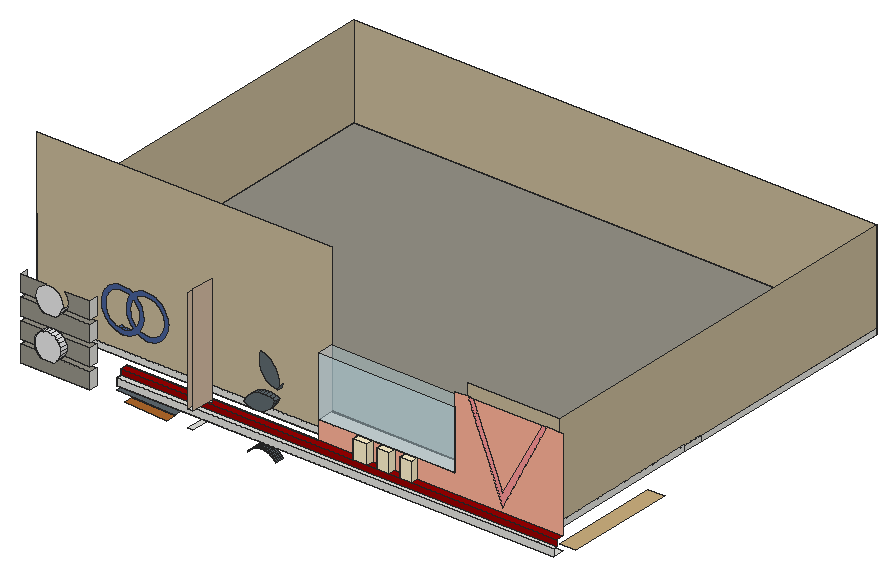
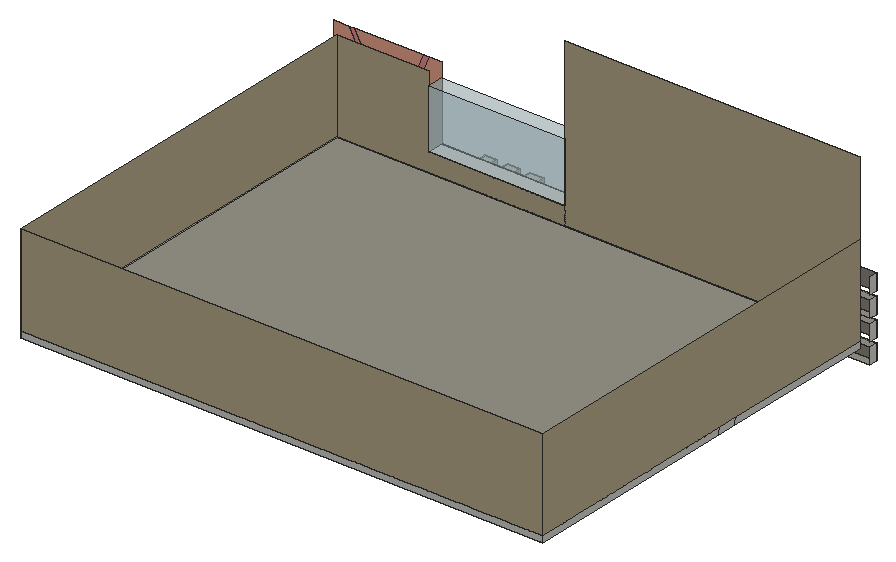
# SketchUp Ruby script. Lengths in inches.
U = 1.inch
M = Sketchup.active_model
def pt(a) = Geom::Point3d.new(a.map { |v| v * U })
def face(e, loops, mat)
  f = e.add_face(loops[0].map { |a| pt(a) })
  loops[1..].each { |l| e.add_face(l.map { |a| pt(a) }).erase! }
  f.material = f.back_material = mat if mat
  f
end
# faces: each face lists its corners as indices into pts; further lists are holes
def faces(e, pts, list, mat = nil) = list.each { |f| face(e, (f[0].is_a?(Array) ? f : [f]).map { |l| l.map { |i| pts[i] } }, mat) }
# xy, xz, yz: faces in a plane at the given z, y or x. An outline is a flat list of corners, or four numbers for a rectangle; further outlines are holes
def ring(l) = l.size == 4 ? [[l[0], l[1]], [l[2], l[1]], [l[2], l[3]], [l[0], l[3]]] : l.each_slice(2).to_a
def flat(e, list, mat, &to3) = list.each { |f| face(e, (f[0].is_a?(Array) ? f : [f]).map { |l| ring(l).map { |u, v| to3.(u, v) } }, mat) }
def xy(e, z, list, mat = nil) = flat(e, list, mat) { |x, y| [x, y, z] }
def xz(e, y, list, mat = nil) = flat(e, list, mat) { |x, z| [x, y, z] }
def yz(e, x, list, mat = nil) = flat(e, list, mat) { |y, z| [x, y, z] }
def lines(e, pts, list) = list.each { |a, b| e.add_line(pt(pts[a]), pt(pts[b])) }
# prism: a flat outline (further loops are holes) pulled along v
def prism(e, loops, v, mat = nil)
  f = face(e, loops, mat); d = Geom::Vector3d.new(v.map { |x| x * U })
  f.pushpull(f.normal.samedirection?(d) ? d.length : -d.length)
end
def box(e, o, s, mat = nil) = prism(e, [[o, [o[0] + s[0], o[1], o[2]], [o[0] + s[0], o[1] + s[1], o[2]], [o[0], o[1] + s[1], o[2]]]], [0, 0, s[2]], mat)
def at(x, y, z, deg = 0) = Geom::Transformation.translation(pt([x, y, z])) * Geom::Transformation.rotation(ORIGIN, Z_AXIS, deg.degrees)
def axes(o, x, y, z) = Geom::Transformation.new([*x, 0, *y, 0, *z, 0, *pt(o).to_a, 1])
def part(name) = M.definitions.add(name)
# library, detail: a bought-in or finely detailed component or shape, given as its bounding box
def library(name, o, s) = part(name).tap { |d| box(d.entities, o, s) }
def detail(e, o, s) = box(e.add_group.entities, o, s)
def put(e, d, t, mat = nil) = e.add_instance(d, t).tap { |i| i.material = mat if mat }
def group(e, t, mat = nil) = e.add_group.tap { |g| g.transformation = t; g.material = mat if mat }.entities
root = M.entities
M.materials.add("[Color A02]").color = [255, 153, 153]
M.materials.add("[Color A07]").color = [153, 0, 0]
M.materials.add("[Color B02]").color = [255, 178, 153]
M.materials.add("[Color D01]").color = [255, 242, 204]
M.materials.add("[Formica Blue]").color = [71, 97, 152]
M.materials.add("[Formica Graystone]").color = [149, 146, 135]
M.materials.add("[Formica Laminate Light]").color = [213, 189, 164]
M.materials.add("[Formica Speckled Grey]").color = [94, 105, 111]
M.materials.add("[Polished Concrete Old]").color = [229, 229, 229]
M.materials.add("[Quartz Light Brown]").color = [199, 184, 152]
M.materials.add("[Translucent Glass Safety]").color = [204, 235, 244]
M.materials["[Translucent Glass Safety]"].alpha = 0.5
M.materials.add("[Wood Bamboo]").color = [177, 105, 43]
M.materials.add("[Wood Floor Light]").color = [204, 176, 127]
xy(root,237.71,[[205.21,257.39,307.34,269.01]],"[Formica Graystone]")
xy(root,241.92,[[424.62,250.56,360.2,253.39,360.79,266.8125,425.21,263.99]],"[Wood Bamboo]")
xy(root,242.2,[[724.72,520.41,868.85,550.03]])
xy(root,251.7,[[963.43,293.12,987.53,454.16]],"[Wood Floor Light]")
xy(root,253.37,[[436.06,250.0625,436.64,263.49,349.35,267.3125,348.76,253.89]],"[Formica Speckled Grey]")
xy(root,258.72,[[479.36,228.58,480.8,261.55,473.4,261.88,471.96,228.91]])
xy(root,259.36,[[491.29,256.01,630.73,269.01]])
xy(root,261.0625,[[963.43,252.2,987.53,269.01]])
xy(root,261.0625,[[350.6,252.2,350.6,269.01,630.73,269.01,630.73,293.12,963.43,293.12,963.43,252.2]],"[Formica Graystone]")
xy(root,261.71,[[205.21,257.39,307.34,269.01]],"[Formica Graystone]")
xy(root,261.71,[[246.96,246.45,260.84,257.39]],"[Polished Concrete Old]")
xy(root,271.3125,[[350.6,252.2,963.43,258.7],[963.43,252.2,987.53,258.7],[350.6,258.7,350.6,269.01,630.73,269.01,630.73,293.12,963.43,293.12,963.43,258.7],[200.82,520.41,963.43,550.03],[200.82,550.03,963.43,870.85]])
xy(root,271.3125,[[200.82,293.12,963.43,520.41]],"[Formica Graystone]")
xy(root,280.3125,[[350.6,258.7,689.3,269.01],[709.64,258.7,724.04,269.01],[742.55,258.7,757.83,269.01],[774.67,258.7,987.53,269.01]],"[Color A07]")
xy(root,280.3125,[[200.82,293.12,963.43,870.85]],"[Formica Graystone]")
xy(root,283.43,[[479.36,228.58,471.96,228.91,473.4,261.88,480.8,261.55]])
xy(root,292.33,[[205.21,257.39,307.34,269.01]],"[Formica Graystone]")
xy(root,298.96,[[205.21,257.39,307.34,269.01]],"[Formica Graystone]")
xy(root,307.55,[[630.73,269.01,829.97,293.12]])
xy(root,307.55,[[689.3,258.7,709.64,269.01],[724.04,258.7,742.55,269.01],[757.83,258.7,774.67,269.01]],"[Color D01]")
xy(root,318.84,[[556.52,261.14,561.09,269.01]],"[Formica Speckled Grey]")
xy(root,322.96,[[205.21,257.39,307.34,269.01]],"[Formica Graystone]")
xy(root,322.96,[[248.17,246.45,264.38,257.39]],"[Polished Concrete Old]")
xz(root,246.45,[[246.96,261.71,260.84,261.71,263.58,262.84,267.59,265.92,269.4375,268.33,270.66,269.93,272.59,274.6,273.25,279.61,272.59,284.61,270.66,289.28,268.32,292.33,267.59,293.29,263.58,296.37,258.91,298.3,253.9,298.96,248.89,298.3,244.22,296.37,240.21,293.29,239.48,292.33,237.14,289.28,235.21,284.61,234.55,279.61,235.21,274.6,237.14,269.93,238.36,268.33,240.21,265.92,244.22,262.84],[248.17,322.96,264.38,322.96,266.07,323.66,270.125,326.77,272.28,329.58,273.24,330.83,275.19,335.55,275.86,340.62,275.19,345.69,273.24,350.42,270.81,353.58,270.125,354.47,266.07,357.59,261.34,359.54,256.27,360.21,251.2,359.54,246.48,357.59,242.42,354.47,241.74,353.58,239.3125,350.42,237.35,345.69,236.6875,340.62,237.35,335.55,239.3125,330.83,240.27,329.58,242.42,326.77,246.48,323.66]],"[Polished Concrete Old]")
xz(root,252.2,[[350.6,261.0625,987.53,271.3125]])
xz(root,257.39,[[253.9,260.25,258.91,260.91,260.84,261.71,246.96,261.71,248.89,260.91],[239.48,292.33,240.21,293.29,244.22,296.37,248.89,298.3,253.9,298.96,258.91,298.3,263.58,296.37,267.59,293.29,268.32,292.33],[256.27,321.04,261.34,321.7,264.38,322.96,248.17,322.96,251.2,321.7]])
xz(root,257.39,[[205.21,237.71,307.34,237.71,307.34,261.71,260.84,261.71,258.91,260.91,253.9,260.25,248.89,260.91,246.96,261.71,205.21,261.71],[205.21,268.33,238.36,268.33,237.14,269.93,235.21,274.6,234.55,279.61,235.21,284.61,237.14,289.28,239.48,292.33,205.21,292.33],[269.4375,268.33,307.34,268.33,307.34,292.33,268.32,292.33,270.66,289.28,272.59,284.61,273.25,279.61,272.59,274.6,270.66,269.93],[205.21,298.96,307.34,298.96,307.34,322.96,264.38,322.96,261.34,321.7,256.27,321.04,251.2,321.7,248.17,322.96,205.21,322.96],[205.21,329.58,240.27,329.58,239.3125,330.83,237.35,335.55,236.6875,340.62,237.35,345.69,239.3125,350.42,241.74,353.58,205.21,353.58],
  [272.28,329.58,307.34,329.58,307.34,353.58,270.81,353.58,273.24,350.42,275.19,345.69,275.86,340.62,275.19,335.55,273.24,330.83]],"[Formica Graystone]")
xz(root,258.7,[[350.6,271.3125,987.53,280.3125]],"[Color A07]")
xz(root,258.7,[[689.3,280.3125,709.64,307.55],[724.04,280.3125,742.55,307.55],[757.83,280.3125,774.67,307.55]],"[Color D01]")
xz(root,261.14,[[545.83,293.67,550.5625,294.15,555.16,295.36,559.51,297.28,563.5,299.84,567.05,303,570.07,306.68,572.47,310.77,574.21,315.2,570.02,317,565.61,318.22,561.09,318.84,556.52,318.84,551.99,318.23,547.59,317.02,543.39,315.23,539.47,312.89,535.9,310.04,532.74,306.74,530.06,303.04,527.89,299.02,532.01,296.64,536.44,294.93,541.09,293.93],[577.86,330.87,578.89,335.32,579.32,339.87,579.125,344.43,578.32,348.93,576.92,353.28,574.95,357.4,572.4375,361.21,569.4375,364.66,566,367.67,562.19,370.19,558.08,372.18,553.74,373.59,552.125,369.125,551.23,364.46,551.07,359.71,551.65,354.99,552.96,350.42,554.97,346.12,557.62,342.17,560.86,338.69,564.59,335.76,568.74,333.44,573.2,331.8]],"[Formica Speckled Grey]")
xz(root,269.01,[[350.6,271.3125,630.73,280.3125]])
xz(root,269.01,[[900.03,286.39,963.43,414.1875,957.83,414.1875,900.03,306.49,897.72,312.17,856.24,414.1875,848.44,414.1875]],"[Color A02]")
xz(root,269.01,[[630.73,280.3125,689.3,307.55],[709.64,280.3125,724.04,307.55],[742.55,280.3125,757.83,307.55],[774.67,280.3125,987.53,280.3125,987.53,414.1875,963.43,414.1875,900.03,286.39,848.44,414.1875,829.97,414.1875,829.97,307.55,774.67,307.55],[900.03,306.49,957.83,414.1875,856.24,414.1875,897.72,312.17]],"[Color B02]")
xz(root,269.01,[[630.73,307.55,829.97,394.11]],"[Translucent Glass Safety]")
xz(root,293.12,[[200.82,271.3125,630.73,280.3125],[630.73,271.3125,963.43,280.3125]])
xz(root,293.12,[[630.73,261.0625,963.43,271.3125]],"[Formica Graystone]")
xz(root,293.12,[[200.82,280.3125,630.73,522.12],[630.73,280.3125,630.73,307.55,829.97,307.55,829.97,414.1875,963.43,414.1875,963.43,280.3125]],"[Quartz Light Brown]")
xz(root,293.12,[[630.73,307.55,829.97,394.11]],"[Translucent Glass Safety]")
xz(root,870.85,[[200.82,271.3125,963.43,280.3125]])
xz(root,870.85,[[200.82,280.3125,963.43,414.1875]],"[Quartz Light Brown]")
yz(root,200.82,[[293.12,271.3125,520.41,280.3125],[520.41,271.3125,550.03,280.3125],[550.03,271.3125,870.85,280.3125]])
yz(root,200.82,[[293.12,280.3125,870.85,414.1875]],"[Quartz Light Brown]")
yz(root,205.21,[[257.39,237.71,269.01,261.71],[257.39,268.33,269.01,292.33],[257.39,298.96,269.01,322.96],[257.39,329.58,269.01,353.58]])
yz(root,307.34,[[257.39,237.71,269.01,261.71],[257.39,268.33,269.01,292.33],[257.39,298.96,269.01,322.96],[257.39,329.58,269.01,353.58]])
yz(root,350.6,[[252.2,261.0625,269.01,271.3125],[258.7,271.3125,269.01,280.3125]])
yz(root,630.73,[[269.01,271.3125,293.12,280.3125],[269.01,307.55,293.12,394.11]])
yz(root,689.3,[[258.7,280.3125,269.01,307.55]],"[Color D01]")
yz(root,709.64,[[258.7,280.3125,269.01,307.55]],"[Color D01]")
yz(root,724.04,[[258.7,280.3125,269.01,307.55]],"[Color D01]")
yz(root,742.55,[[258.7,280.3125,269.01,307.55]],"[Color D01]")
yz(root,757.83,[[258.7,280.3125,269.01,307.55]],"[Color D01]")
yz(root,774.67,[[258.7,280.3125,269.01,307.55]],"[Color D01]")
yz(root,829.97,[[269.01,307.55,293.12,394.11]])
yz(root,963.43,[[293.12,271.3125,520.41,280.3125],[520.41,271.3125,550.03,280.3125],[550.03,271.3125,870.85,280.3125]])
yz(root,963.43,[[293.12,280.3125,870.85,414.1875]],"[Quartz Light Brown]")
p = [[537.87,269.01,238.18],[538.6,269.01,239.24],[538.6,256.01,239.24],[537.87,256.01,238.18],[578.55,269.01,239.24],[579.28,269.01,238.18],
  [579.28,256.01,238.18],[578.55,256.01,239.24],[539.39,269.01,240.27],[539.39,256.01,240.27],[577.76,269.01,240.27],[577.76,256.01,240.27],
  [540.23,269.01,241.25],[540.23,256.01,241.25],[576.92,269.01,241.25],[576.92,256.01,241.25],[541.12,269.01,242.1875],[541.12,256.01,242.1875],
  [576.03,269.01,242.1875],[576.03,256.01,242.1875],[542.06,269.01,243.08],[542.06,256.01,243.08],[575.1,269.01,243.08],[575.1,256.01,243.08],
  [543.04,269.01,243.92],[543.04,256.01,243.92],[574.11,269.01,243.92],[574.11,256.01,243.92],[544.07,269.01,244.7],[544.07,256.01,244.7],
  [573.09,269.01,244.7],[573.09,256.01,244.7],[545.13,269.01,245.4375],[545.13,256.01,245.4375],[572.02,269.01,245.4375],[572.02,256.01,245.4375],
  [546.23,269.01,246.11],[546.23,256.01,246.11],[570.92,269.01,246.11],[570.92,256.01,246.11],[547.37,269.01,246.73],[547.37,256.01,246.73],
  [569.79,269.01,246.73],[569.79,256.01,246.73],[548.54,269.01,247.28],[548.54,256.01,247.28],[568.62,269.01,247.28],[568.62,256.01,247.28],
  [549.73,269.01,247.78],[549.73,256.01,247.78],[567.42,269.01,247.78],[567.42,256.01,247.78],[550.95,269.01,248.21],[550.95,256.01,248.21],
  [566.21,269.01,248.21],[566.21,256.01,248.21],[552.1875,269.01,248.58],[552.1875,256.01,248.58],[564.97,269.01,248.58],[564.97,256.01,248.58],
  [553.44,269.01,248.88],[553.44,256.01,248.88],[563.71,269.01,248.88],[563.71,256.01,248.88],[554.72,269.01,249.11],[554.72,256.01,249.11],
  [562.4375,269.01,249.11],[562.4375,256.01,249.11],[556,269.01,249.28],[556,256.01,249.28],[561.16,269.01,249.28],[561.16,256.01,249.28],
  [557.29,269.01,249.38],[557.29,256.01,249.38],[559.87,269.01,249.38],[559.87,256.01,249.38],[558.58,269.01,249.42],[558.58,256.01,249.42],
  [473.4,261.88,283.43],[473.4,261.88,258.72],[480.8,261.55,258.72],[480.8,261.55,283.43],[244.22,257.39,262.84],[246.96,257.39,261.71],
  [246.96,246.45,261.71],[244.22,246.45,262.84],[260.84,257.39,261.71],[263.58,257.39,262.84],[263.58,246.45,262.84],[260.84,246.45,261.71],
  [240.21,257.39,265.92],[240.21,246.45,265.92],[267.59,257.39,265.92],[267.59,246.45,265.92],[238.36,257.39,268.33],[238.36,246.45,268.33],
  [269.4375,257.39,268.33],[269.4375,246.45,268.33],[237.14,257.39,269.93],[237.14,246.45,269.93],[270.66,257.39,269.93],[270.66,246.45,269.93],
  [235.21,257.39,274.6],[235.21,246.45,274.6],[272.59,257.39,274.6],[272.59,246.45,274.6],[234.55,257.39,279.61],[234.55,246.45,279.61],
  [273.25,257.39,279.61],[273.25,246.45,279.61],[235.21,257.39,284.61],[235.21,246.45,284.61],[272.59,257.39,284.61],[272.59,246.45,284.61],
  [480.8,261.55,442.52],[479.36,228.58,442.52],[479.36,228.58,283.43],[473.4,261.88,435.11],[471.96,228.91,283.43],[471.96,228.91,435.11],
  [237.14,257.39,289.28],[237.14,246.45,289.28],[270.66,257.39,289.28],[270.66,246.45,289.28],[240.21,257.39,293.29],[239.48,257.39,292.33],
  [239.48,246.45,292.33],[240.21,246.45,293.29],[268.32,257.39,292.33],[267.59,257.39,293.29],[267.59,246.45,293.29],[268.32,246.45,292.33],
  [244.22,257.39,296.37],[244.22,246.45,296.37],[263.58,257.39,296.37],[263.58,246.45,296.37],[541.09,269.01,293.93],[545.83,269.01,293.67],
  [545.83,261.14,293.67],[541.09,261.14,293.93],[550.5625,269.01,294.15],[550.5625,261.14,294.15],[536.44,269.01,294.93],[536.44,261.14,294.93],
  [555.16,269.01,295.36],[555.16,261.14,295.36],[532.01,269.01,296.64],[532.01,261.14,296.64],[559.51,269.01,297.28],[559.51,261.14,297.28],
  [248.89,257.39,298.3],[248.89,246.45,298.3],[258.91,257.39,298.3],[258.91,246.45,298.3],[527.89,269.01,299.02],[527.89,261.14,299.02],
  [563.5,269.01,299.84],[563.5,261.14,299.84],[253.9,257.39,298.96],[253.9,246.45,298.96],[530.06,269.01,303.04],[530.06,261.14,303.04],
  [567.05,269.01,303],[567.05,261.14,303],[532.74,269.01,306.74],[532.74,261.14,306.74],[570.07,269.01,306.68],[570.07,261.14,306.68],
  [535.9,269.01,310.04],[535.9,261.14,310.04],[572.47,269.01,310.77],[572.47,261.14,310.77],[539.47,269.01,312.89],[539.47,261.14,312.89],
  [574.21,269.01,315.2],[574.21,261.14,315.2],[543.39,269.01,315.23],[543.39,261.14,315.23],[547.59,269.01,317.02],[547.59,261.14,317.02],
  [570.02,269.01,317],[570.02,261.14,317],[551.99,269.01,318.23],[551.99,261.14,318.23],[565.61,269.01,318.22],[565.61,261.14,318.22],
  [556.52,269.01,318.84],[556.52,261.14,318.84],[561.09,269.01,318.84],[561.09,261.14,318.84],[246.48,257.39,323.66],[248.17,257.39,322.96],
  [248.17,246.45,322.96],[246.48,246.45,323.66],[264.38,257.39,322.96],[266.07,257.39,323.66],[266.07,246.45,323.66],[264.38,246.45,322.96],
  [242.42,257.39,326.77],[242.42,246.45,326.77],[270.125,257.39,326.77],[270.125,246.45,326.77],[240.27,257.39,329.58],[240.27,246.45,329.58],
  [272.28,257.39,329.58],[272.28,246.45,329.58],[239.3125,257.39,330.83],[239.3125,246.45,330.83],[273.24,257.39,330.83],[273.24,246.45,330.83],
  [379.1,253,338.44],[379.2,252.99,338.55],[379.91,252.96,338.12],[382.91,252.83,336.71],[386.03,252.69,335.63],[389.25,252.55,334.88],
  [392.53,252.41,334.47],[395.84,252.26,334.41],[399.14,252.12,334.69],[402.38,251.98,335.32],[405.55,251.84,336.28],[408.59,251.71,337.57],
  [411.49,251.58,339.17],[414.2,251.46,341.0625],[416.7,251.35,343.23],[418.96,251.25,345.65],[420.95,251.16,348.29],[422.66,251.09,351.125],
  [424.0625,251.03,354.12],[425.14,250.98,357.25],[425.89,250.95,360.48],[426.3,250.93,363.76],[426.36,250.93,367.07],[426.08,250.9375,370.37],
  [425.46,250.97,373.62],[424.49,251.01,376.79],[423.21,251.06,379.83],[421.61,251.13,382.73],[419.71,251.22,385.45],[417.55,251.3125,387.95],
  [415.13,251.42,390.21],[412.5,251.53,392.21],[409.66,251.66,393.92],[406.67,251.79,395.32],[403.54,251.93,396.4],[400.32,252.07,397.15],
  [397.04,252.21,397.56],[393.73,252.36,397.62],[390.4375,252.5,397.34],[387.19,252.64,396.71],[384.03,252.78,395.75],[380.98,252.92,394.46],
  [378.09,253.04,392.86],[375.375,253.16,390.97],[372.875,253.27,388.8],[372.78,253.27,388.7],[372.07,253.31,389.13],[369.07,253.4375,390.53],
  [365.95,253.57,391.61],[362.72,253.72,392.36],[359.44,253.86,392.77],[356.14,254,392.84],[352.84,254.15,392.55],[349.59,254.29,391.93],
  [346.43,254.43,390.96],[343.38,254.5625,389.67],[340.49,254.69,388.07],[337.78,254.81,386.18],[335.28,254.92,384.01],[333.02,255.02,381.59],
  [331.02,255.1,378.95],[329.32,255.18,376.12],[327.91,255.24,373.12],[326.83,255.29,369.99],[326.08,255.32,366.77],[325.67,255.34,363.48],
  [325.61,255.34,360.17],[325.9,255.33,356.875],[326.52,255.3,353.625],[327.48,255.26,350.46],[328.77,255.2,347.41],[330.37,255.13,344.51],
  [332.26,255.05,341.8],[334.43,254.96,339.3],[336.84,254.85,337.03],[339.48,254.73,335.04],[342.3125,254.61,333.33],[345.31,254.48,331.92],
  [348.43,254.34,330.84],[351.65,254.2,330.09],[354.9375,254.06,329.68],[358.24,253.91,329.62],[361.54,253.77,329.9],[364.78,253.625,330.53],
  [367.95,253.49,331.49],[371,253.35,332.78],[373.89,253.23,334.38],[376.6,253.11,336.28],[374.44,253.2,341.82],[374.51,253.2,341.77],
  [373.21,253.26,340.64],[370.97,253.35,339.07],[368.58,253.46,337.75],[366.07,253.57,336.6875],[363.46,253.68,335.89],[360.78,253.8,335.375],
  [358.06,253.92,335.14],[355.33,254.04,335.19],[352.62,254.16,335.53],[349.96,254.27,336.15],[347.38,254.39,337.04],[344.91,254.5,338.2],
  [342.57,254.6,339.61],[340.4,254.69,341.26],[338.4,254.78,343.125],[336.62,254.86,345.19],[335.05,254.93,347.43],[333.73,254.99,349.82],
  [332.67,255.03,352.34],[331.88,255.07,354.95],[331.36,255.09,357.64],[331.13,255.1,360.36],[331.18,255.1,363.09],[331.52,255.08,365.8],
  [332.13,255.06,368.46],[333.03,255.02,371.04],[334.18,254.97,373.52],[335.59,254.9,375.86],[337.24,254.83,378.04],[339.1,254.75,380.03],
  [341.17,254.66,381.82],[343.41,254.5625,383.38],[345.79,254.46,384.71],[348.31,254.35,385.77],[350.92,254.23,386.5625],[353.6,254.12,387.08],
  [356.32,254,387.32],[359.05,253.875,387.26],[361.76,253.76,386.93],[364.42,253.64,386.31],[367,253.53,385.41],[369.13,253.43,384.41],
  [368.62,253.46,383.74],[366.91,253.53,380.91],[365.51,253.59,377.91],[364.43,253.64,374.78],[363.68,253.67,371.56],[363.27,253.69,368.27],
  [363.21,253.69,364.96],[363.49,253.68,361.66],[364.12,253.65,358.41],[365.08,253.61,355.25],[366.37,253.56,352.2],[367.97,253.49,349.3],
  [369.86,253.4,346.58],[372.03,253.31,344.08],[384.98,252.74,341.83],[382.85,252.83,342.83],[383.35,252.8125,343.5],[385.0625,252.74,346.34],
  [386.46,252.67,349.34],[387.55,252.63,352.46],[388.3,252.59,355.6875],[388.7,252.58,358.97],[388.77,252.57,362.28],[388.48,252.59,365.58],
  [387.86,252.61,368.83],[386.9,252.66,372],[385.61,252.71,375.05],[384.01,252.78,377.95],[382.12,252.87,380.66],[379.95,252.96,383.16],
  [377.54,253.07,385.42],[377.46,253.07,385.48],[378.77,253.01,386.61],[381,252.91,388.17],[383.39,252.81,389.49],[385.91,252.7,390.56],
  [388.52,252.58,391.35],[391.2,252.47,391.87],[393.92,252.35,392.1],[396.65,252.23,392.05],[399.36,252.11,391.71],[402.01,251.99,391.09],
  [404.59,251.88,390.2],[407.07,251.77,389.04],[409.4,251.67,387.63],[411.58,251.57,385.98],[413.57,251.49,384.12],[415.36,251.41,382.05],
  [416.92,251.34,379.8125],[418.24,251.28,377.42],[419.3,251.24,374.9],[420.1,251.2,372.29],[420.62,251.18,369.61],[420.85,251.17,366.89],
  [420.8,251.17,364.15],[420.46,251.19,361.44],[419.84,251.21,358.78],[418.95,251.25,356.2],[417.79,251.3,353.73],[416.38,251.36,351.39],
  [414.74,251.4375,349.21],[412.87,251.52,347.21],[410.81,251.61,345.42],[408.57,251.71,343.86],[406.18,251.8125,342.54],[403.67,251.92,341.47],
  [401.06,252.04,340.68],[398.375,252.15,340.16],[395.66,252.27,339.93],[392.93,252.39,339.98],[390.22,252.51,340.32],[387.5625,252.625,340.9375],
  [378.78,253.01,346.6],[378.23,253.04,345.87],[377.99,253.05,346.05],[376,253.13,347.91],[374.21,253.21,349.98],[372.65,253.28,352.22],
  [371.33,253.34,354.61],[370.27,253.38,357.125],[369.48,253.42,359.74],[368.96,253.44,362.42],[368.73,253.45,365.15],[368.78,253.45,367.875],
  [369.11,253.44,370.59],[369.73,253.41,373.25],[370.625,253.37,375.83],[371.78,253.32,378.3],[373.19,253.26,380.64],[373.74,253.23,381.375],
  [373.98,253.22,381.2],[375.98,253.13,379.33],[377.76,253.06,377.27],[379.32,252.99,375.03],[380.64,252.93,372.63],[381.71,252.88,370.12],
  [382.5,252.85,367.5],[383.02,252.83,364.82],[383.25,252.82,362.1],[383.2,252.82,359.37],[382.86,252.83,356.66],[382.24,252.86,353.99],
  [381.35,252.9,351.41],[380.19,252.95,348.9375],[358.8125,266.9,329.62],[362.11,266.75,329.9],[355.51,267.04,329.68],[352.22,267.1875,330.09],
  [365.35,266.61,330.53],[349,267.33,330.84],[368.52,266.47,331.49],[237.35,257.39,335.55],[237.35,246.45,335.55],[275.19,257.39,335.55],
  [275.19,246.45,335.55],[345.88,267.47,331.92],[573.2,269.01,331.8],[577.86,269.01,330.87],[577.86,261.14,330.87],[573.2,261.14,331.8],
  [578.89,269.01,335.32],[578.89,261.14,335.32]]
faces(root,p,[[0,1,2,3],[4,5,6,7],[1,8,9,2],[10,4,7,11],[8,12,13,9],[14,10,11,15],[12,16,17,13],[18,14,15,19],
  [16,20,21,17],[22,18,19,23],[20,24,25,21],[26,22,23,27],[24,28,29,25],[30,26,27,31],[28,32,33,29],[34,30,31,35],
  [32,36,37,33],[38,34,35,39],[36,40,41,37],[42,38,39,43],[40,44,45,41],[46,42,43,47],[44,48,49,45],[50,46,47,51],
  [48,52,53,49],[54,50,51,55],[52,56,57,53],[58,54,55,59],[56,60,61,57],[62,58,59,63],[60,64,65,61],[66,62,63,67],
  [64,68,69,65],[70,66,67,71],[68,72,73,69],[74,70,71,75],[72,76,77,73],[76,74,75,77],[136,137,138,139],[137,140,141,138],
  [142,136,139,143],[140,144,145,141],[146,142,143,147],[144,148,149,145],[154,146,147,155],[148,156,157,149],[160,154,155,161],[156,162,163,157],
  [164,160,161,165],[162,166,167,163],[168,164,165,169],[166,170,171,167],[172,168,169,173],[170,174,175,171],[176,172,173,177],[178,176,177,179],
  [174,180,181,175],[182,178,179,183],[180,184,185,181],[186,182,183,187],[184,188,189,185],[458,459,460,461],[459,462,463,460]],"[Formica Speckled Grey]")
faces(root,p,[[78,79,80,81],[82,83,84,85],[90,82,85,91],[94,90,91,95]])
faces(root,p,[[86,87,88,89],[87,92,93,88],[92,96,97,93],[98,94,95,99],[96,100,101,97],[102,98,99,103],[100,104,105,101],[106,102,103,107],
  [104,108,109,105],[110,106,107,111],[108,112,113,109],[120,110,111,121],[112,122,123,113],[124,125,120,121,126,127],[122,128,129,130,131,123],[132,124,127,133],
  [129,134,135,130],[150,132,133,151],[134,152,153,135],[158,150,151,159],[152,158,159,153],[190,191,192,193],[194,195,196,197],[198,190,193,199],
  [195,200,201,196],[202,198,199,203],[200,204,205,201],[206,202,203,207],[204,208,209,205],[453,206,207,454],[208,455,456,209]],"[Polished Concrete Old]")
faces(root,p,[[81,114,115,116],[117,78,118,119]],"[Formica Laminate Light]")
faces(root,p,[[[210,211,212,213,214,215,216,217,218,219,220,221,222,223,224,225,226,227,228,229,230,231,232,233,234,235,236,237,238,239,240,241,242,243,244,245,246,247,248,249,250,251,252,253,254,255,256,257,258,259,260,261,262,263,264,265,266,267,268,269,270,271,272,273,274,275,276,277,278,279,280,281,282,283,284,285,286,287,288,289,290,291,292,293,294,295,296,297],[298,299,300,301,302,303,304,305,306,307,308,309,310,311,312,313,314,315,316,317,318,319,320,321,322,323,324,325,326,327,328,329,330,331,332,333,334,335,336,337,338,339,340,341,342,343,344,345,346,347,348,349,350,351,352,353,354,355],[356,357,358,359,360,361,362,363,364,365,366,367,368,369,370,371,372,373,374,375,376,377,378,379,380,381,382,383,384,385,386,387,388,389,390,391,392,393,394,395,396,397,398,399,400,401,402,403,404,405,406,407,408,409,410,411,412,413],[414,415,416,417,418,419,420,421,422,423,424,425,426,427,428,429,430,431,432,433,434,435,436,437,438,439,440,441,442,443,444,445]],[446,447,292,291],[448,446,291,290],[449,448,290,289],[447,450,293,292],[451,449,289,288],[450,452,294,293],[457,451,288,287]],"[Formica Blue]")
